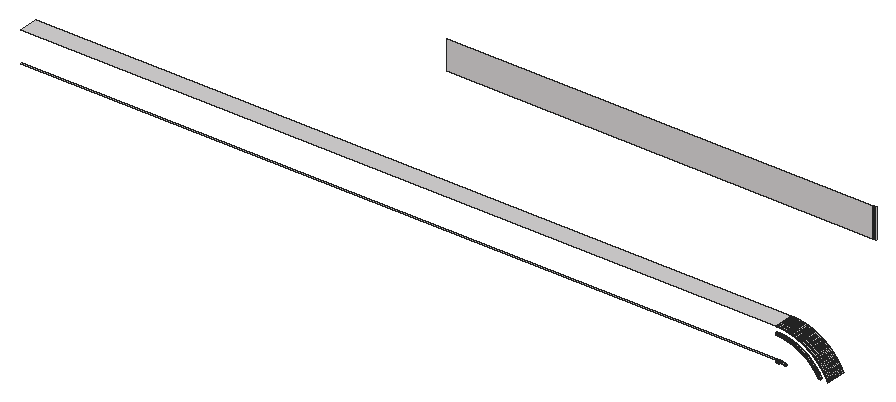
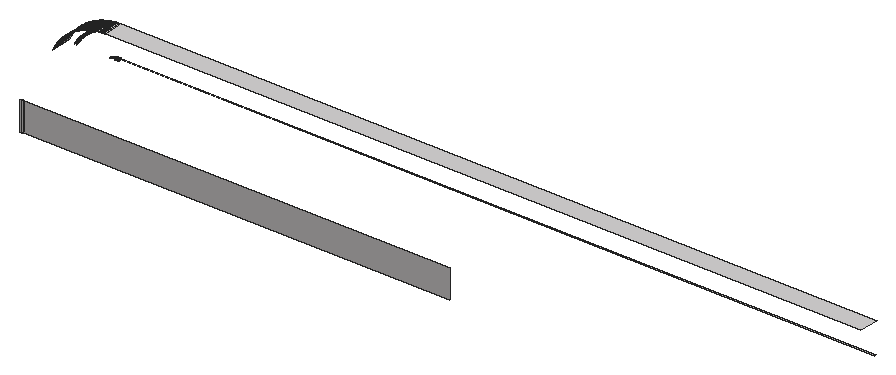
# SketchUp Ruby script. Lengths in inches.
U = 1.inch
M = Sketchup.active_model
def pt(a) = Geom::Point3d.new(a.map { |v| v * U })
def face(e, loops, mat)
  f = e.add_face(loops[0].map { |a| pt(a) })
  loops[1..].each { |l| e.add_face(l.map { |a| pt(a) }).erase! }
  f.material = f.back_material = mat if mat
  f
end
# faces: each face lists its corners as indices into pts; further lists are holes
def faces(e, pts, list, mat = nil) = list.each { |f| face(e, (f[0].is_a?(Array) ? f : [f]).map { |l| l.map { |i| pts[i] } }, mat) }
# xy, xz, yz: faces in a plane at the given z, y or x. An outline is a flat list of corners, or four numbers for a rectangle; further outlines are holes
def ring(l) = l.size == 4 ? [[l[0], l[1]], [l[2], l[1]], [l[2], l[3]], [l[0], l[3]]] : l.each_slice(2).to_a
def flat(e, list, mat, &to3) = list.each { |f| face(e, (f[0].is_a?(Array) ? f : [f]).map { |l| ring(l).map { |u, v| to3.(u, v) } }, mat) }
def xy(e, z, list, mat = nil) = flat(e, list, mat) { |x, y| [x, y, z] }
def xz(e, y, list, mat = nil) = flat(e, list, mat) { |x, z| [x, y, z] }
def yz(e, x, list, mat = nil) = flat(e, list, mat) { |y, z| [x, y, z] }
def lines(e, pts, list) = list.each { |a, b| e.add_line(pt(pts[a]), pt(pts[b])) }
# prism: a flat outline (further loops are holes) pulled along v
def prism(e, loops, v, mat = nil)
  f = face(e, loops, mat); d = Geom::Vector3d.new(v.map { |x| x * U })
  f.pushpull(f.normal.samedirection?(d) ? d.length : -d.length)
end
def box(e, o, s, mat = nil) = prism(e, [[o, [o[0] + s[0], o[1], o[2]], [o[0] + s[0], o[1] + s[1], o[2]], [o[0], o[1] + s[1], o[2]]]], [0, 0, s[2]], mat)
def at(x, y, z, deg = 0) = Geom::Transformation.translation(pt([x, y, z])) * Geom::Transformation.rotation(ORIGIN, Z_AXIS, deg.degrees)
def axes(o, x, y, z) = Geom::Transformation.new([*x, 0, *y, 0, *z, 0, *pt(o).to_a, 1])
def part(name) = M.definitions.add(name)
# library, detail: a bought-in or finely detailed component or shape, given as its bounding box
def library(name, o, s) = part(name).tap { |d| box(d.entities, o, s) }
def detail(e, o, s) = box(e.add_group.entities, o, s)
def put(e, d, t, mat = nil) = e.add_instance(d, t).tap { |i| i.material = mat if mat }
def group(e, t, mat = nil) = e.add_group.tap { |g| g.transformation = t; g.material = mat if mat }.entities
root = M.entities
M.materials.add("[Quartz Light Brown]").color = [215, 212, 212]
xy(root,99.98,[[504.75,38,504.88,39]],"[Quartz Light Brown]")
xy(root,99.99,[[504.5,38,504.63,39]],"[Quartz Light Brown]")
xy(root,100,[[503.96,38,504.125,39],[504.125,38,504.25,39],[504.25,38,504.375,39]],"[Quartz Light Brown]")
xy(root,100.97,[[504.93,38,505.07,39]],"[Quartz Light Brown]")
xy(root,100.99,[[504.53,38,504.67,39]],"[Quartz Light Brown]")
xy(root,101,[[36.04,38,503.96,39],[503.96,38,504.13,39],[504.13,38,504.27,39],[504.27,38,504.4,39]],"[Quartz Light Brown]")
xy(root,114.98,[[504.97,38,505.22,39]],"[Quartz Light Brown]")
xy(root,115,[[503.99,38,504.24,39],[504.24,38,504.49,39]],"[Quartz Light Brown]")
xy(root,115.98,[[505.01,38,505.26,39]],"[Quartz Light Brown]")
xy(root,116,[[503.99,38,504.25,39],[504.25,38,504.5,39]],"[Quartz Light Brown]")
xy(root,120,[[36,38,504,50],[504,38,504.28,50],[504.28,38,504.57,50]],"[Quartz Light Brown]")
xz(root,143,[[216,114,480,132],[480,114,480.2,132]],"[Quartz Light Brown]")
xz(root,143.01,[[480.39,114,480.59,132]],"[Quartz Light Brown]")
p = [[506.13,39,99.86],[506.13,38,99.86],[506.25,38,99.84],[506.25,39,99.84],[506.38,38,99.82],[506.38,39,99.82],
  [506.5,38,99.8],[506.5,39,99.8],[506.625,38,99.78],[506.625,39,99.78],[506.75,38,99.76],[506.75,39,99.76],
  [510.13,38,99.85],[510.13,39,99.85],[510.26,39,99.81],[510.26,38,99.81],[530.56,39,99.99],[530.56,38,99.99],
  [530.68,38,99.78],[530.68,39,99.78],[536.2,38,100.09],[536.33,38,99.84],[536.33,50,99.84],[536.2,50,100.09],
  [505.26,39,99.95],[505.26,38,99.95],[505.38,38,99.94],[505.38,39,99.94],[505.51,38,99.93],[505.51,39,99.93],
  [505.63,38,99.92],[505.63,39,99.92],[505.76,38,99.9],[505.76,39,99.9],[505.88,38,99.89],[505.88,39,99.89],
  [506.01,38,99.875],[506.01,39,99.875],[509.76,38,99.99],[509.76,39,99.99],[509.88,39,99.95],[509.88,38,99.95],
  [510.01,39,99.9],[510.01,38,99.9],[531.67,38,100.07],[531.67,39,100.07],[531.8,39,99.85],[531.8,38,99.85],
  [504.375,39,100],[504.375,38,100],[504.5,38,99.99],[504.5,39,99.99],[504.63,39,99.99],[504.63,38,99.99],
  [504.75,38,99.98],[504.75,39,99.98],[504.88,39,99.98],[504.88,38,99.98],[505,38,99.97],[505,39,99.97],
  [505.13,38,99.96],[505.13,39,99.96],[509.51,38,100.08],[509.51,39,100.08],[509.63,39,100.04],[509.63,38,100.04],
  [530.43,39,100.2],[530.43,38,100.2],[509.25,38,100.17],[509.25,39,100.17],[509.38,39,100.125],[509.38,38,100.125],
  [531.54,38,100.29],[531.54,39,100.29],[536.08,38,100.34],[536.08,50,100.34],[508.87,38,100.29],[508.87,39,100.29],
  [509,39,100.25],[509,38,100.25],[509.125,39,100.21],[509.125,38,100.21],[530.3,39,100.4],[530.3,38,100.4],
  [508.61,38,100.36],[508.61,39,100.36],[508.74,39,100.32],[508.74,38,100.32],[531.41,38,100.51],[531.41,39,100.51],
  [535.95,38,100.6],[535.95,50,100.6],[508.23,38,100.47],[508.23,39,100.47],[508.36,39,100.43],[508.36,38,100.43],
  [508.49,39,100.4],[508.49,38,100.4],[530.17,39,100.61],[530.17,38,100.61],[507.84,38,100.5625],[507.84,39,100.5625],
  [507.97,39,100.53],[507.97,38,100.53],[508.1,39,100.5],[508.1,38,100.5],[531.28,38,100.72],[531.28,39,100.72],
  [507.32,38,100.67],[507.32,39,100.67],[507.45,39,100.65],[507.45,38,100.65],[507.58,39,100.62],[507.58,38,100.62],
  [507.71,39,100.59],[507.71,38,100.59],[530.04,39,100.82],[530.04,38,100.82],[535.82,38,100.85],[535.82,50,100.85],
  [506.79,38,100.77],[506.79,39,100.77],[506.92,39,100.75],[506.92,38,100.75],[507.05,39,100.72],[507.05,38,100.72],
  [507.19,39,100.7],[507.19,38,100.7],[531.15,38,100.93],[531.15,39,100.93],[506.13,38,100.87],[506.13,39,100.87],
  [506.26,39,100.85],[506.26,38,100.85],[506.4,39,100.83],[506.4,38,100.83],[506.53,39,100.8125],[506.53,38,100.8125],
  [506.66,39,100.79],[506.66,38,100.79],[529.91,39,101.02],[529.91,38,101.02],[535.68,38,101.09],[535.68,50,101.09],
  [505.2,38,100.96],[505.2,39,100.96],[505.33,39,100.95],[505.33,38,100.95],[505.47,39,100.9375],[505.47,38,100.9375],
  [505.6,39,100.92],[505.6,38,100.92],[505.73,39,100.91],[505.73,38,100.91],[505.87,39,100.9],[505.87,38,100.9],
  [506,39,100.88],[506,38,100.88],[531.02,38,101.15],[531.02,39,101.15],[504.4,38,101],[504.4,39,101],
  [504.53,39,100.99],[504.53,38,100.99],[504.67,38,100.99],[504.67,39,100.99],[504.8,39,100.98],[504.8,38,100.98],
  [504.93,39,100.97],[504.93,38,100.97],[505.07,38,100.97],[505.07,39,100.97],[529.78,39,101.22],[529.78,38,101.22],
  [530.88,38,101.36],[530.88,39,101.36],[535.55,38,101.34],[535.55,50,101.34],[529.64,39,101.42],[529.64,38,101.42],
  [535.41,38,101.59],[535.41,50,101.59],[529.5,39,101.625],[529.5,38,101.625],[530.75,38,101.57],[530.75,39,101.57],
  [529.36,39,101.83],[529.36,38,101.83],[530.61,38,101.78],[530.61,39,101.78],[535.27,38,101.84],[535.27,50,101.84],
  [529.22,39,102.02],[529.22,38,102.02],[530.47,38,101.99],[530.47,39,101.99],[535.13,38,102.08],[535.13,50,102.08],
  [529.08,39,102.22],[529.08,38,102.22],[530.32,38,102.19],[530.32,39,102.19],[534.99,38,102.33],[534.99,50,102.33],
  [528.9375,39,102.42],[528.9375,38,102.42],[530.18,38,102.4],[530.18,39,102.4],[534.84,38,102.57],[534.84,50,102.57],
  [528.79,39,102.61],[528.79,38,102.61],[530.04,38,102.61],[530.04,39,102.61],[528.64,39,102.81],[528.64,38,102.81],
  [529.89,38,102.81],[529.89,39,102.81],[534.7,38,102.81],[534.7,50,102.81],[528.49,39,103],[528.49,38,103],
  [529.74,38,103.01],[529.74,39,103.01],[534.55,38,103.05],[534.55,50,103.05],[528.34,39,103.19],[528.34,38,103.19],
  [529.59,38,103.21],[529.59,39,103.21],[534.4,38,103.29],[534.4,50,103.29],[528.19,39,103.38],[528.19,38,103.38],
  [529.4375,38,103.41],[529.4375,39,103.41],[534.24,38,103.53],[534.24,50,103.53],[528.04,39,103.57],[528.04,38,103.57],
  [529.28,38,103.61],[529.28,39,103.61],[534.09,38,103.76],[534.09,50,103.76],[527.89,39,103.76],[527.89,38,103.76],
  [529.13,38,103.8125],[529.13,39,103.8125],[527.73,39,103.95],[527.73,38,103.95],[528.97,38,104.01],[528.97,39,104.01],
  [533.93,38,104],[533.93,50,104],[527.57,39,104.13],[527.57,38,104.13],[528.82,38,104.2],[528.82,39,104.2],
  [533.77,38,104.24],[533.77,50,104.24],[527.41,39,104.32],[527.41,38,104.32],[528.66,38,104.4],[528.66,39,104.4],
  [533.62,38,104.47],[533.62,50,104.47],[527.25,39,104.5],[527.25,38,104.5],[528.5,38,104.59],[528.5,39,104.59],
  [527.09,39,104.68],[527.09,38,104.68],[533.45,38,104.7],[533.45,50,104.7],[528.33,38,104.78],[528.33,39,104.78],
  [526.93,39,104.86],[526.93,38,104.86],[533.29,38,104.93],[533.29,50,104.93],[528.17,38,104.97],[528.17,39,104.97],
  [526.76,39,105.04],[526.76,38,105.04],[533.125,38,105.16],[533.125,50,105.16],[526.6,39,105.22],[526.6,38,105.22],
  [528,38,105.16],[528,39,105.16],[526.43,39,105.4],[526.43,38,105.4],[527.84,38,105.35],[527.84,39,105.35],
  [532.96,38,105.39],[532.96,50,105.39],[527.67,38,105.54],[527.67,39,105.54],[526.26,39,105.57],[526.26,38,105.57],
  [532.79,38,105.62],[532.79,50,105.62],[527.5,38,105.72],[527.5,39,105.72],[526.09,39,105.75],[526.09,38,105.75],
  [532.62,38,105.84],[532.62,50,105.84],[525.92,39,105.92],[525.92,38,105.92],[527.33,38,105.91],[527.33,39,105.91],
  [532.45,38,106.06],[532.45,50,106.06],[525.75,39,106.09],[525.75,38,106.09],[527.15,38,106.09],[527.15,39,106.09],
  [525.57,39,106.26],[525.57,38,106.26],[526.98,38,106.27],[526.98,39,106.27],[532.27,38,106.29],[532.27,50,106.29],
  [525.4,39,106.43],[525.4,38,106.43],[526.8,38,106.45],[526.8,39,106.45],[532.1,38,106.51],[532.1,50,106.51],
  [525.22,39,106.6],[525.22,38,106.6],[526.63,38,106.63],[526.63,39,106.63],[531.92,38,106.73],[531.92,50,106.73],
  [525.04,39,106.76],[525.04,38,106.76],[526.45,38,106.8],[526.45,39,106.8],[531.74,38,106.95],[531.74,50,106.95],
  [524.86,39,106.93],[524.86,38,106.93],[526.27,38,106.98],[526.27,39,106.98],[524.68,39,107.09],[524.68,38,107.09],
  [531.56,38,107.16],[531.56,50,107.16],[526.09,38,107.15],[526.09,39,107.15],[524.5,39,107.25],[524.5,38,107.25],
  [525.91,38,107.33],[525.91,39,107.33],[531.375,38,107.38],[531.375,50,107.38],[524.32,39,107.41],[524.32,38,107.41],
  [525.72,38,107.5],[525.72,39,107.5],[524.13,39,107.57],[524.13,38,107.57],[531.19,38,107.59],[531.19,50,107.59],
  [525.54,38,107.67],[525.54,39,107.67],[523.95,39,107.73],[523.95,38,107.73],[531,38,107.81],[531,50,107.81],
  [523.76,39,107.89],[523.76,38,107.89],[525.35,38,107.84],[525.35,39,107.84],[525.16,38,108],[525.16,39,108],
  [530.82,38,108.02],[530.82,50,108.02],[523.57,39,108.04],[523.57,38,108.04],[523.38,39,108.19],[523.38,38,108.19],
  [524.97,38,108.17],[524.97,39,108.17],[530.625,38,108.23],[530.625,50,108.23],[523.19,39,108.34],[523.19,38,108.34],
  [524.78,38,108.33],[524.78,39,108.33],[530.4375,38,108.4375],[530.4375,50,108.4375],[523,39,108.49],[523,38,108.49],
  [524.59,38,108.5],[524.59,39,108.5],[530.24,38,108.64],[530.24,50,108.64],[522.81,39,108.64],[522.81,38,108.64],
  [524.4,38,108.66],[524.4,39,108.66],[522.61,39,108.79],[522.61,38,108.79],[530.05,38,108.85],[530.05,50,108.85],
  [524.2,38,108.82],[524.2,39,108.82],[522.42,39,108.9375],[522.42,38,108.9375],[524.01,38,108.97],[524.01,39,108.97],
  [529.85,38,109.05],[529.85,50,109.05],[522.22,39,109.08],[522.22,38,109.08],[523.8125,38,109.13],[523.8125,39,109.13],
  [522.02,39,109.22],[522.02,38,109.22],[523.61,38,109.28],[523.61,39,109.28],[529.65,38,109.26],[529.65,50,109.26],
  [521.83,39,109.36],[521.83,38,109.36],[523.41,38,109.4375],[523.41,39,109.4375],[529.46,38,109.46],[529.46,50,109.46],
  [521.625,39,109.5],[521.625,38,109.5],[523.21,38,109.59],[523.21,39,109.59],[521.42,39,109.64],[521.42,38,109.64],
  [529.26,38,109.65],[529.26,50,109.65],[521.22,39,109.78],[521.22,38,109.78],[523.01,38,109.74],[523.01,39,109.74],
  [522.81,38,109.89],[522.81,39,109.89],[529.05,38,109.85],[529.05,50,109.85],[521.02,39,109.91],[521.02,38,109.91],
  [520.82,39,110.04],[520.82,38,110.04],[522.61,38,110.04],[522.61,39,110.04],[528.85,38,110.05],[528.85,50,110.05],
  [520.61,39,110.17],[520.61,38,110.17],[522.4,38,110.18],[522.4,39,110.18],[528.64,38,110.24],[528.64,50,110.24],
  [520.4,39,110.3],[520.4,38,110.3],[522.19,38,110.32],[522.19,39,110.32],[528.4375,38,110.4375],[528.4375,50,110.4375],
  [520.2,39,110.43],[520.2,38,110.43],[521.99,38,110.47],[521.99,39,110.47],[519.99,39,110.56],[519.99,38,110.56],
  [528.23,38,110.625],[528.23,50,110.625],[521.78,38,110.61],[521.78,39,110.61],[519.78,39,110.68],[519.78,38,110.68],
  [521.57,38,110.75],[521.57,39,110.75],[528.02,38,110.82],[528.02,50,110.82],[519.57,39,110.81],[519.57,38,110.81],
  [521.36,38,110.88],[521.36,39,110.88],[519.36,39,110.93],[519.36,38,110.93],[527.81,38,111],[527.81,50,111],
  [519.15,39,111.05],[519.15,38,111.05],[521.15,38,111.02],[521.15,39,111.02],[518.93,39,111.17],[518.93,38,111.17],
  [520.93,38,111.15],[520.93,39,111.15],[527.59,38,111.19],[527.59,50,111.19],[518.72,39,111.28],[518.72,38,111.28],
  [520.72,38,111.28],[520.72,39,111.28],[527.38,38,111.375],[527.38,50,111.375],[518.51,39,111.4],[518.51,38,111.4],
  [520.51,38,111.41],[520.51,39,111.41],[518.29,39,111.51],[518.29,38,111.51],[520.29,38,111.54],[520.29,39,111.54],
  [527.16,38,111.56],[527.16,50,111.56],[518.07,39,111.62],[518.07,38,111.62],[520.07,38,111.67],[520.07,39,111.67],
  [517.86,39,111.73],[517.86,38,111.73],[526.95,38,111.74],[526.95,50,111.74],[517.64,39,111.84],[517.64,38,111.84],
  [519.85,38,111.8],[519.85,39,111.8],[526.73,38,111.92],[526.73,50,111.92],[517.42,39,111.95],[517.42,38,111.95],
  [519.64,38,111.92],[519.64,39,111.92],[517.2,39,112.05],[517.2,38,112.05],[519.42,38,112.04],[519.42,39,112.04],
  [526.51,38,112.1],[526.51,50,112.1],[516.98,39,112.15],[516.98,38,112.15],[519.2,38,112.16],[519.2,39,112.16],
  [526.29,38,112.27],[526.29,50,112.27],[516.76,39,112.25],[516.76,38,112.25],[518.97,38,112.28],[518.97,39,112.28],
  [516.53,39,112.35],[516.53,38,112.35],[518.75,38,112.4],[518.75,39,112.4],[526.06,38,112.45],[526.06,50,112.45],
  [516.3125,39,112.45],[516.3125,38,112.45],[518.53,38,112.51],[518.53,39,112.51],[525.84,38,112.62],[525.84,50,112.62],
  [515.86,39,112.64],[515.86,38,112.64],[516.09,38,112.55],[516.09,39,112.55],[518.3,38,112.625],[518.3,39,112.625],
  [515.64,39,112.73],[515.64,38,112.73],[518.08,38,112.74],[518.08,39,112.74],[525.62,38,112.79],[525.62,50,112.79],
  [515.41,39,112.82],[515.41,38,112.82],[517.85,38,112.85],[517.85,39,112.85],[515.19,39,112.91],[515.19,38,112.91],
  [517.625,38,112.95],[517.625,39,112.95],[525.39,38,112.96],[525.39,50,112.96],[514.96,39,113],[514.96,38,113],
  [514.73,39,113.08],[514.73,38,113.08],[517.4,38,113.0625],[517.4,39,113.0625],[525.16,38,113.125],[525.16,50,113.125],
  [514.5,39,113.17],[514.5,38,113.17],[517.17,38,113.16],[517.17,39,113.16],[524.93,38,113.29],[524.93,50,113.29],
  [514.04,39,113.33],[514.04,38,113.33],[514.27,38,113.25],[514.27,39,113.25],[516.9375,38,113.27],[516.9375,39,113.27],
  [513.8125,39,113.41],[513.8125,38,113.41],[516.71,38,113.37],[516.71,39,113.37],[524.7,38,113.45],[524.7,50,113.45],
  [513.58,39,113.48],[513.58,38,113.48],[516.48,38,113.47],[516.48,39,113.47],[513.35,39,113.56],[513.35,38,113.56],
  [516.25,38,113.5625],[516.25,39,113.5625],[524.47,38,113.62],[524.47,50,113.62],[512.88,39,113.7],[512.88,38,113.7],
  [513.12,38,113.63],[513.12,39,113.63],[516.01,38,113.66],[516.01,39,113.66],[524.24,38,113.77],[524.24,50,113.77],
  [512.65,39,113.77],[512.65,38,113.77],[515.78,38,113.75],[515.78,39,113.75],[512.18,39,113.9],[512.18,38,113.9],
  [512.41,38,113.84],[512.41,39,113.84],[515.3125,38,113.93],[515.3125,39,113.93],[515.55,39,113.84],[515.55,38,113.84],
  [524,38,113.93],[524,50,113.93],[511.94,39,113.96],[511.94,38,113.96],[515.08,38,114.02],[515.08,39,114.02],
  [523.76,38,114.09],[523.76,50,114.09],[511.47,39,114.09],[511.47,38,114.09],[511.71,38,114.03],[511.71,39,114.03],
  [514.84,38,114.11],[514.84,39,114.11],[480.2,143,132],[480.2,143,114],[480.39,143.01,114],[480.39,143.01,132],
  [480.59,143.01,132],[480.59,143.01,114],[480.79,143.02,114],[480.79,143.02,132],[480.98,143.03,114],[480.98,143.03,132],
  [481.18,143.05,114],[481.18,143.05,132],[481.37,143.0625,114],[481.37,143.0625,132],[481.57,143.08,114],[481.57,143.08,132],
  [481.76,143.1,114],[481.76,143.1,132],[481.96,143.13,114],[481.96,143.13,132],[482.15,143.16,114],[482.15,143.16,132],
  [511,39,114.2],[511,38,114.2],[511.24,38,114.14],[511.24,39,114.14],[514.6,38,114.19],[514.6,39,114.19],
  [523.53,38,114.24],[523.53,50,114.24],[510.76,39,114.25],[510.76,38,114.25],[514.37,38,114.27],[514.37,39,114.27],
  [523.29,38,114.4],[523.29,50,114.4],[510.29,39,114.36],[510.29,38,114.36],[510.52,38,114.31],[510.52,39,114.31],
  [514.13,38,114.36],[514.13,39,114.36],[509.81,39,114.45],[509.81,38,114.45],[510.05,38,114.4],[510.05,39,114.4],
  [513.65,38,114.51],[513.65,39,114.51],[513.89,39,114.43],[513.89,38,114.43],[523.05,38,114.55],[523.05,50,114.55],
  [509.09,39,114.58],[509.09,38,114.58],[509.33,38,114.54],[509.33,39,114.54],[509.57,38,114.5],[509.57,39,114.5],
  [513.41,38,114.59],[513.41,39,114.59],[522.81,38,114.7],[522.81,50,114.7],[508.61,39,114.66],[508.61,38,114.66],
  [508.85,38,114.62],[508.85,39,114.62],[513.17,38,114.66],[513.17,39,114.66],[507.89,39,114.76],[507.89,38,114.76],
  [508.125,38,114.72],[508.125,39,114.72],[508.37,38,114.69],[508.37,39,114.69],[512.6875,38,114.8],[512.6875,39,114.8],
  [512.93,39,114.73],[512.93,38,114.73],[522.57,38,114.84],[522.57,50,114.84],[506.92,39,114.86],[506.92,38,114.86],
  [507.16,38,114.84],[507.16,39,114.84],[507.4,38,114.8125],[507.4,39,114.8125],[507.64,38,114.79],[507.64,39,114.79],
  [512.44,38,114.87],[512.44,39,114.87],[522.33,38,114.99],[522.33,50,114.99],[505.7,39,114.95],[505.7,38,114.95],
  [505.95,38,114.9375],[505.95,39,114.9375],[506.1875,38,114.92],[506.1875,39,114.92],[506.43,38,114.9],[506.43,39,114.9],
  [506.67,38,114.88],[506.67,39,114.88],[511.96,38,114.99],[511.96,39,114.99],[512.2,39,114.93],[512.2,38,114.93],
  [504.49,39,115],[504.49,38,115],[504.73,38,114.99],[504.73,39,114.99],[504.97,38,114.98],[504.97,39,114.98],
  [505.22,39,114.98],[505.22,38,114.98],[505.46,38,114.97],[505.46,39,114.97],[511.71,38,115.06],[511.71,39,115.06],
  [522.08,38,115.13],[522.08,50,115.13],[511.23,38,115.17],[511.23,39,115.17],[511.47,39,115.12],[511.47,38,115.12],
  [521.84,38,115.27],[521.84,50,115.27],[510.74,38,115.28],[510.74,39,115.28],[510.98,39,115.23],[510.98,38,115.23],
  [510.24,38,115.39],[510.24,39,115.39],[510.49,39,115.34],[510.49,38,115.34],[521.59,38,115.41],[521.59,50,115.41],
  [509.75,38,115.48],[509.75,39,115.48],[510,39,115.43],[510,38,115.43],[521.34,38,115.55],[521.34,50,115.55],
  [509.25,38,115.57],[509.25,39,115.57],[509.5,39,115.52],[509.5,38,115.52],[521.09,38,115.68],[521.09,50,115.68],
  [508.51,38,115.68],[508.51,39,115.68],[508.76,39,115.64],[508.76,38,115.64],[509.01,39,115.61],[509.01,38,115.61],
  [507.76,38,115.78],[507.76,39,115.78],[508.01,39,115.75],[508.01,38,115.75],[508.26,39,115.72],[508.26,38,115.72],
  [520.85,38,115.82],[520.85,50,115.82],[507.01,38,115.86],[507.01,39,115.86],[507.26,39,115.83],[507.26,38,115.83],
  [507.51,39,115.81],[507.51,38,115.81],[520.6,38,115.95],[520.6,50,115.95],[505.76,38,115.95],[505.76,39,115.95],
  [506.01,39,115.9375],[506.01,38,115.9375],[506.26,39,115.92],[506.26,38,115.92],[506.51,39,115.9],[506.51,38,115.9],
  [506.76,39,115.88],[506.76,38,115.88],[520.34,38,116.08],[520.34,50,116.08],[504.5,38,116],[504.5,39,116],
  [504.75,39,115.99],[504.75,38,115.99],[505.01,39,115.98],[505.01,38,115.98],[505.26,38,115.98],[505.26,39,115.98],
  [505.51,39,115.96],[505.51,38,115.96],[520.09,38,116.2],[520.09,50,116.2],[519.84,38,116.33],[519.84,50,116.33],
  [519.58,38,116.45],[519.58,50,116.45],[519.33,38,116.57],[519.33,50,116.57],[519.07,38,116.69],[519.07,50,116.69],
  [518.81,38,116.8125],[518.81,50,116.8125],[518.56,38,116.93],[518.56,50,116.93],[518.3,38,117.04],[518.3,50,117.04],
  [518.04,38,117.15],[518.04,50,117.15],[517.78,38,117.26],[517.78,50,117.26],[517.51,38,117.37],[517.51,50,117.37],
  [517.25,38,117.47],[517.25,50,117.47],[516.99,38,117.58],[516.99,50,117.58],[516.73,38,117.68],[516.73,50,117.68],
  [516.46,38,117.77],[516.46,50,117.77],[516.19,38,117.87],[516.19,50,117.87],[515.93,38,117.97],[515.93,50,117.97],
  [515.66,38,118.06],[515.66,50,118.06],[515.125,38,118.24],[515.39,38,118.15],[515.39,50,118.15],[515.125,50,118.24],
  [514.86,38,118.32],[514.86,50,118.32],[514.59,38,118.41],[514.59,50,118.41],[514.31,38,118.49],[514.31,50,118.49],
  [514.04,38,118.57],[514.04,50,118.57],[513.5,38,118.72],[513.77,38,118.65],[513.77,50,118.65],[513.5,50,118.72],
  [513.23,38,118.8],[513.23,50,118.8],[512.95,38,118.87],[512.95,50,118.87],[512.4,38,119.01],[512.68,38,118.9375],
  [512.68,50,118.9375],[512.4,50,119.01],[512.13,38,119.07],[512.13,50,119.07],[511.58,38,119.19],[511.85,38,119.13],
  [511.85,50,119.13],[511.58,50,119.19],[511.3,38,119.25],[511.3,50,119.25],[510.75,38,119.36],[511.02,38,119.31],
  [511.02,50,119.31],[510.75,50,119.36],[510.1875,38,119.46],[510.47,38,119.41],[510.47,50,119.41],[510.1875,50,119.46],
  [509.63,38,119.56],[509.91,38,119.51],[509.91,50,119.51],[509.63,50,119.56],[508.79,38,119.68],[509.07,38,119.64],
  [509.07,50,119.64],[508.79,50,119.68],[509.35,38,119.6],[509.35,50,119.6],[508.23,38,119.75],[508.51,38,119.72],
  [508.51,50,119.72],[508.23,50,119.75],[507.11,38,119.87],[507.39,38,119.84],[507.39,50,119.84],[507.11,50,119.87],
  [507.67,38,119.8125],[507.67,50,119.8125],[507.95,38,119.78],[507.95,50,119.78],[505.7,38,119.96],[505.98,38,119.95],
  [505.98,50,119.95],[505.7,50,119.96],[506.26,38,119.93],[506.26,50,119.93],[506.54,38,119.91],[506.54,50,119.91],
  [506.82,38,119.89],[506.82,50,119.89],[504.57,38,120],[504.85,38,119.99],[504.85,50,119.99],[504.57,50,120],
  [505.13,38,119.98],[505.13,50,119.98],[505.41,38,119.97],[505.41,50,119.97]]
faces(root,p,[[0,1,2,3],[3,2,4,5],[5,4,6,7],[7,6,8,9],[9,8,10,11],[12,13,14,15],[16,17,18,19],[20,21,22,23],
  [24,25,26,27],[27,26,28,29],[29,28,30,31],[31,30,32,33],[33,32,34,35],[35,34,36,37],[37,36,1,0],[38,39,40,41],
  [41,40,42,43],[43,42,13,12],[44,45,46,47],[48,49,50,51],[52,53,54,55],[56,57,58,59],[59,58,60,61],[61,60,25,24],
  [62,63,64,65],[65,64,39,38],[66,67,17,16],[68,69,70,71],[71,70,63,62],[72,73,45,44],[74,20,23,75],[76,77,78,79],
  [79,78,80,81],[81,80,69,68],[82,83,67,66],[84,85,86,87],[87,86,77,76],[88,89,73,72],[90,74,75,91],[92,93,94,95],
  [95,94,96,97],[97,96,85,84],[98,99,83,82],[100,101,102,103],[103,102,104,105],[105,104,93,92],[106,107,89,88],[108,109,110,111],
  [111,110,112,113],[113,112,114,115],[115,114,101,100],[116,117,99,98],[118,90,91,119],[120,121,122,123],[123,122,124,125],[125,124,126,127],
  [127,126,109,108],[128,129,107,106],[130,131,132,133],[133,132,134,135],[135,134,136,137],[137,136,138,139],[139,138,121,120],[140,141,117,116],
  [142,118,119,143],[144,145,146,147],[147,146,148,149],[149,148,150,151],[151,150,152,153],[153,152,154,155],[155,154,156,157],[157,156,131,130],
  [158,159,129,128],[160,161,162,163],[164,165,166,167],[167,166,168,169],[170,171,145,144],[172,173,141,140],[174,175,159,158],[176,142,143,177],
  [178,179,173,172],[180,176,177,181],[182,183,179,178],[184,185,175,174],[186,187,183,182],[188,189,185,184],[190,180,181,191],[192,193,187,186],
  [194,195,189,188],[196,190,191,197],[198,199,193,192],[200,201,195,194],[202,196,197,203],[204,205,199,198],[206,207,201,200],[208,202,203,209],
  [210,211,205,204],[212,213,207,206],[214,215,211,210],[216,217,213,212],[218,208,209,219],[220,221,215,214],[222,223,217,216],[224,218,219,225],
  [226,227,221,220],[228,229,223,222],[230,224,225,231],[232,233,227,226],[234,235,229,228],[236,230,231,237],[238,239,233,232],[240,241,235,234],
  [242,236,237,243],[244,245,239,238],[246,247,241,240],[248,249,245,244],[250,251,247,246],[252,242,243,253],[254,255,249,248],[256,257,251,250],
  [258,252,253,259],[260,261,255,254],[262,263,257,256],[264,258,259,265],[266,267,261,260],[268,269,263,262],[270,271,267,266],[272,264,265,273],
  [274,275,269,268],[276,277,271,270],[278,272,273,279],[280,281,275,274],[282,283,277,276],[284,278,279,285],[286,287,283,282],[288,289,281,280],
  [290,291,287,286],[292,293,289,288],[294,284,285,295],[296,297,293,292],[298,299,291,290],[300,294,295,301],[302,303,297,296],[304,305,299,298],
  [306,300,301,307],[308,309,305,304],[310,311,303,302],[312,306,307,313],[314,315,309,308],[316,317,311,310],[318,319,315,314],[320,321,317,316],
  [322,312,313,323],[324,325,319,318],[326,327,321,320],[328,322,323,329],[330,331,325,324],[332,333,327,326],[334,328,329,335],[336,337,331,330],
  [338,339,333,332],[340,334,335,341],[342,343,337,336],[344,345,339,338],[346,347,343,342],[348,340,341,349],[350,351,345,344],[352,353,347,346],
  [354,355,351,350],[356,348,349,357],[358,359,353,352],[360,361,355,354],[362,363,359,358],[364,356,357,365],[366,367,361,360],[368,369,363,362],
  [370,364,365,371],[372,373,369,368],[374,375,367,366],[376,377,375,374],[378,370,371,379],[380,381,373,372],[382,383,381,380],[384,385,377,376],
  [386,378,379,387],[388,389,383,382],[390,391,385,384],[392,386,387,393],[394,395,389,388],[396,397,391,390],[398,392,393,399],[400,401,395,394],
  [402,403,397,396],[404,405,401,400],[406,398,399,407],[408,409,403,402],[410,411,405,404],[412,413,409,408],[414,406,407,415],[416,417,411,410],
  [418,419,413,412],[420,421,417,416],[422,423,419,418],[424,414,415,425],[426,427,421,420],[428,429,423,422],[430,424,425,431],[432,433,427,426],
  [434,435,429,428],[436,437,433,432],[438,430,431,439],[440,441,437,436],[442,443,435,434],[444,445,443,442],[446,438,439,447],[448,449,441,440],
  [450,451,449,448],[452,453,445,444],[454,446,447,455],[456,457,451,450],[458,459,453,452],[460,454,455,461],[462,463,457,456],[464,465,459,458],
  [466,460,461,467],[468,469,463,462],[470,471,465,464],[472,473,469,468],[474,466,467,475],[476,477,471,470],[478,479,473,472],[480,481,477,476],
  [482,474,475,483],[484,485,479,478],[486,487,481,480],[488,489,485,484],[490,482,483,491],[492,493,489,488],[494,495,487,486],[496,497,493,492],
  [498,499,495,494],[500,490,491,501],[502,503,497,496],[504,505,499,498],[506,500,501,507],[508,509,503,502],[510,511,505,504],[512,513,509,508],
  [514,515,511,510],[516,506,507,517],[518,519,513,512],[520,521,515,514],[522,523,519,518],[524,516,517,525],[526,527,523,522],[528,529,521,520],
  [530,524,525,531],[532,533,527,526],[534,535,529,528],[536,537,533,532],[538,539,535,534],[540,530,531,541],[542,543,537,536],[544,545,539,538],
  [546,540,541,547],[548,549,543,542],[550,551,545,544],[552,553,549,548],[554,555,551,550],[556,546,547,557],[558,559,553,552],[560,561,555,554],
  [562,556,557,563],[564,565,566,567],[567,566,559,558],[568,569,561,560],[570,571,565,564],[572,573,569,568],[574,562,563,575],[576,577,571,570],
  [578,579,573,572],[580,581,577,576],[582,583,579,578],[584,574,575,585],[586,587,581,580],[588,589,587,586],[590,591,583,582],[592,584,585,593],
  [594,595,589,588],[596,597,591,590],[598,592,593,599],[600,601,602,603],[603,602,595,594],[604,605,597,596],[606,607,601,600],[608,609,605,604],
  [610,598,599,611],[612,613,607,606],[614,615,609,608],[616,617,613,612],[618,619,615,614],[620,610,611,621],[622,623,624,625],[625,624,617,616],
  [626,627,619,618],[628,620,621,629],[630,631,623,622],[632,633,627,626],[634,635,636,637],[637,636,631,630],[638,639,640,641],[641,640,633,632],
  [642,628,629,643],[644,645,635,634],[646,647,639,638],[648,642,643,649],[650,651,652,653],[653,652,645,644],[654,655,647,646],[656,657,658,659],
  [660,661,662,663],[663,662,664,665],[665,664,666,667],[667,666,668,669],[669,668,670,671],[671,670,672,673],[673,672,674,675],[675,674,676,677],
  [678,679,680,681],[681,680,651,650],[682,683,655,654],[684,648,649,685],[686,687,679,678],[688,689,683,682],[690,684,685,691],[692,693,694,695],
  [695,694,687,686],[696,697,689,688],[698,699,700,701],[701,700,693,692],[702,703,704,705],[705,704,697,696],[706,690,691,707],[708,709,710,711],
  [711,710,712,713],[713,712,699,698],[714,715,703,702],[716,706,707,717],[718,719,720,721],[721,720,709,708],[722,723,715,714],[724,725,726,727],
  [727,726,728,729],[729,728,719,718],[730,731,732,733],[733,732,723,722],[734,716,717,735],[736,737,738,739],[739,738,740,741],[741,740,742,743],
  [743,742,725,724],[744,745,731,730],[746,734,735,747],[748,749,750,751],[751,750,752,753],[753,752,754,755],[755,754,756,757],[757,756,737,736],
  [758,759,760,761],[761,760,745,744],[762,763,764,765],[765,764,766,767],[768,769,770,771],[771,770,749,748],[772,773,759,758],[774,746,747,775],
  [776,777,778,779],[779,778,773,772],[780,774,775,781],[782,783,784,785],[785,784,777,776],[786,787,788,789],[789,788,783,782],[790,780,781,791],
  [792,793,794,795],[795,794,787,786],[796,790,791,797],[798,799,800,801],[801,800,793,792],[802,796,797,803],[804,805,806,807],[807,806,808,809],
  [809,808,799,798],[810,811,812,813],[813,812,814,815],[815,814,805,804],[816,802,803,817],[818,819,820,821],[821,820,822,823],[823,822,811,810],
  [824,816,817,825],[826,827,828,829],[829,828,830,831],[831,830,832,833],[833,832,834,835],[835,834,819,818],[836,824,825,837],[838,839,840,841],
  [841,840,842,843],[844,845,846,847],[847,846,827,826],[848,836,837,849],[850,848,849,851],[852,850,851,853],[854,852,853,855],[856,854,855,857],
  [858,856,857,859],[860,858,859,861],[862,860,861,863],[864,862,863,865],[866,864,865,867],[868,866,867,869],[870,868,869,871],[872,870,871,873],
  [874,872,873,875],[876,874,875,877],[878,876,877,879],[880,878,879,881],[882,880,881,883],[884,885,886,887],[885,882,883,886],[888,884,887,889],
  [890,888,889,891],[892,890,891,893],[894,892,893,895],[896,897,898,899],[897,894,895,898],[900,896,899,901],[902,900,901,903],[904,905,906,907],
  [905,902,903,906],[908,904,907,909],[910,911,912,913],[911,908,909,912],[914,910,913,915],[916,917,918,919],[917,914,915,918],[920,921,922,923],
  [921,916,919,922],[924,925,926,927],[925,920,923,926],[928,929,930,931],[929,932,933,930],[932,924,927,933],[934,935,936,937],[935,928,931,936],
  [938,939,940,941],[939,942,943,940],[942,944,945,943],[944,934,937,945],[946,947,948,949],[947,950,951,948],[950,952,953,951],[952,954,955,953],
  [954,938,941,955],[956,957,958,959],[957,960,961,958],[960,962,963,961],[962,946,949,963]],"[Quartz Light Brown]")
